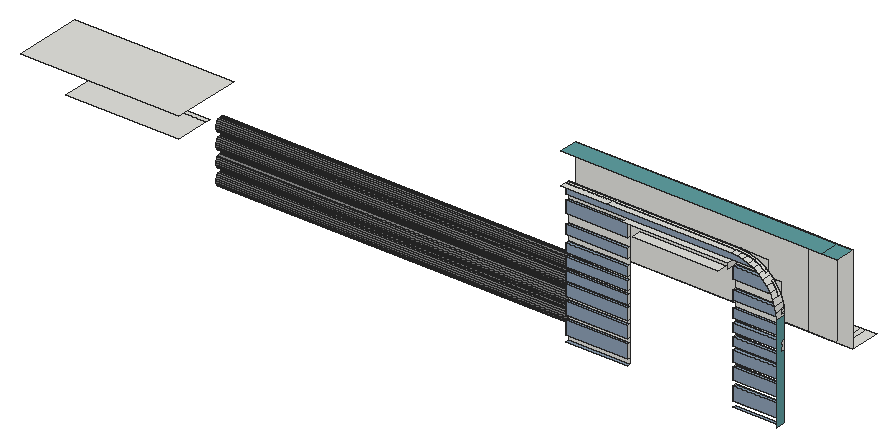
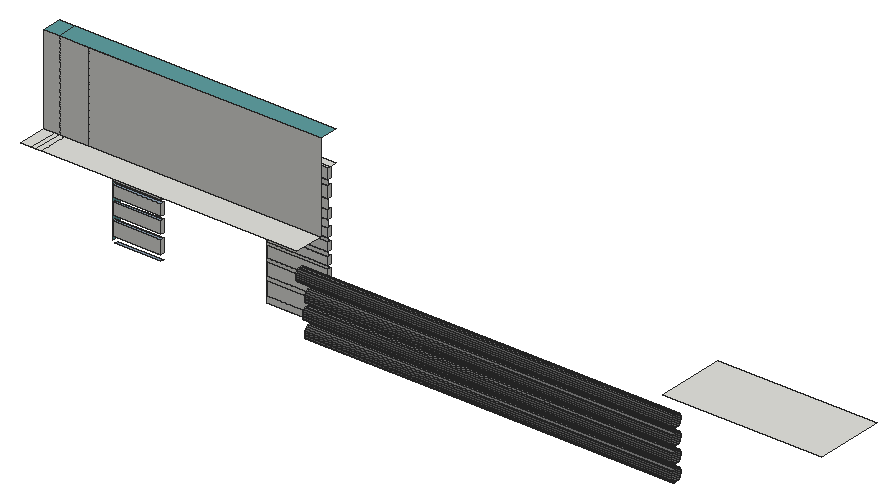
# SketchUp Ruby script. Lengths in inches.
U = 1.inch
M = Sketchup.active_model
def pt(a) = Geom::Point3d.new(a.map { |v| v * U })
def face(e, loops, mat)
  f = e.add_face(loops[0].map { |a| pt(a) })
  loops[1..].each { |l| e.add_face(l.map { |a| pt(a) }).erase! }
  f.material = f.back_material = mat if mat
  f
end
# faces: each face lists its corners as indices into pts; further lists are holes
def faces(e, pts, list, mat = nil) = list.each { |f| face(e, (f[0].is_a?(Array) ? f : [f]).map { |l| l.map { |i| pts[i] } }, mat) }
# xy, xz, yz: faces in a plane at the given z, y or x. An outline is a flat list of corners, or four numbers for a rectangle; further outlines are holes
def ring(l) = l.size == 4 ? [[l[0], l[1]], [l[2], l[1]], [l[2], l[3]], [l[0], l[3]]] : l.each_slice(2).to_a
def flat(e, list, mat, &to3) = list.each { |f| face(e, (f[0].is_a?(Array) ? f : [f]).map { |l| ring(l).map { |u, v| to3.(u, v) } }, mat) }
def xy(e, z, list, mat = nil) = flat(e, list, mat) { |x, y| [x, y, z] }
def xz(e, y, list, mat = nil) = flat(e, list, mat) { |x, z| [x, y, z] }
def yz(e, x, list, mat = nil) = flat(e, list, mat) { |y, z| [x, y, z] }
def lines(e, pts, list) = list.each { |a, b| e.add_line(pt(pts[a]), pt(pts[b])) }
# prism: a flat outline (further loops are holes) pulled along v
def prism(e, loops, v, mat = nil)
  f = face(e, loops, mat); d = Geom::Vector3d.new(v.map { |x| x * U })
  f.pushpull(f.normal.samedirection?(d) ? d.length : -d.length)
end
def box(e, o, s, mat = nil) = prism(e, [[o, [o[0] + s[0], o[1], o[2]], [o[0] + s[0], o[1] + s[1], o[2]], [o[0], o[1] + s[1], o[2]]]], [0, 0, s[2]], mat)
def at(x, y, z, deg = 0) = Geom::Transformation.translation(pt([x, y, z])) * Geom::Transformation.rotation(ORIGIN, Z_AXIS, deg.degrees)
def axes(o, x, y, z) = Geom::Transformation.new([*x, 0, *y, 0, *z, 0, *pt(o).to_a, 1])
def part(name) = M.definitions.add(name)
# library, detail: a bought-in or finely detailed component or shape, given as its bounding box
def library(name, o, s) = part(name).tap { |d| box(d.entities, o, s) }
def detail(e, o, s) = box(e.add_group.entities, o, s)
def put(e, d, t, mat = nil) = e.add_instance(d, t).tap { |i| i.material = mat if mat }
def group(e, t, mat = nil) = e.add_group.tap { |g| g.transformation = t; g.material = mat if mat }.entities
root = M.entities
M.materials.add("[0081_CadetBlue]").color = [95, 158, 160]
M.materials.add("[0110_LightSlateGray]").color = [139, 158, 178]
M.materials.add("[0133_Gray]").color = [128, 128, 128]
xy(root,388.02,[[160.53,8,179.47,9],[211.78,8,225.89,9]],"[0110_LightSlateGray]")
xy(root,389.79,[[160.53,8,179.47,9],[211.78,8,226.5625,9]],"[0110_LightSlateGray]")
xy(root,393.9,[[160.53,8,179.47,9],[211.78,8,226.5625,9]],"[0110_LightSlateGray]")
xy(root,395.43,[[160.53,8,179.47,9],[211.78,8,226.5625,9]],"[0110_LightSlateGray]")
xy(root,399.05,[[160.53,8,179.47,9],[211.78,8,226.5625,9]],"[0110_LightSlateGray]")
xy(root,400.39,[[160.53,8,179.47,9],[211.78,8,226.5625,9]],"[0110_LightSlateGray]")
xy(root,403.8125,[[160.53,8,179.47,9],[211.78,8,226.5625,9]],"[0110_LightSlateGray]")
xy(root,404.77,[[160.53,8,179.47,9],[211.78,8,226.5625,9]],"[0110_LightSlateGray]")
xy(root,407.32,[[160.53,8,179.47,9],[211.78,8,226.5625,9]],"[0110_LightSlateGray]")
xy(root,407.79,[[14,0,48.4375,10.4375],[14,10.4375,48.4375,12]])
xy(root,408.61,[[160.53,8,179.47,9],[211.78,8,226.59,9]],"[0110_LightSlateGray]")
xy(root,411.25,[[160.53,8,179.47,9],[211.78,8,226.59,9]],"[0110_LightSlateGray]")
xy(root,412.46,[[160.53,8,179.47,9],[211.78,8,226.5625,9]],"[0110_LightSlateGray]")
xy(root,414,[[0,0,48.4375,21],[160.53,12,238.75,21],[238.75,12,240.375,21],[240.375,12,241.9375,21],[241.9375,12,245.1875,21]])
xy(root,415.15,[[160.53,8,179.47,9],[211.78,8,226.5625,9]],"[0110_LightSlateGray]")
xy(root,417.42,[[160.53,8,179.47,9],[211.78,8,226.53,9]],"[0110_LightSlateGray]")
xy(root,420.17,[[160.53,8,179.47,9],[211.78,8,226.38,9]],"[0110_LightSlateGray]")
xy(root,423.16,[[160.53,8,179.47,9],[211.78,8,225.55,9]],"[0110_LightSlateGray]")
xy(root,425.29,[[182.53,6,208.72,9]])
xy(root,426.8,[[160.53,8,179.47,9],[211.78,8,223.28,9]],"[0110_LightSlateGray]")
xy(root,428.35,[[179.47,6,211.78,9]])
xy(root,428.36,[[160.53,8,221.7,9]],"[0110_LightSlateGray]")
xy(root,431.57,[[160.53,6,174.8,8],[174.8,6,212.95,8],[160.53,8,174.8,9],[174.8,8,212.95,9]])
xy(root,441.0625,[[160.53,6,240.375,12],[240.375,6,245.1875,12]],"[0081_CadetBlue]")
xz(root,8,[[160.53,389.79,179.47,393.9],[211.78,389.79,226.5625,393.9],[160.53,395.43,179.47,399.05],[211.78,395.43,226.5625,399.05],[160.53,400.39,179.47,403.8125],
  [211.78,400.39,226.5625,403.8125],[160.53,404.77,179.47,407.32],[211.78,404.77,226.5625,407.32],[160.53,408.61,179.47,411.25],[211.78,408.61,226.59,411.25],
  [160.53,412.46,179.47,415.15],[211.78,412.46,226.5625,415.15],[160.53,417.42,179.47,420.17],[211.78,417.42,226.53,417.42,226.53,418.83,226.47,419.72,226.38,420.17,211.78,420.17],[160.53,423.16,179.47,426.8],
  [211.78,423.16,225.55,423.16,224.76,424.76,223.77,426.24,223.28,426.8,211.78,426.8],[160.53,428.36,221.7,428.36,221.25,428.76,219.77,429.75,218.17,430.54,216.48,431.11,214.73,431.46,212.95,431.57,160.53,431.57]],"[0110_LightSlateGray]")
xz(root,9,[[160.53,388.02,179.47,389.79],[160.53,389.79,179.47,393.9],[211.78,389.79,226.5625,393.9],[160.53,393.9,179.47,395.43],[160.53,395.43,179.47,399.05],
  [211.78,395.43,226.5625,399.05],[160.53,399.05,179.47,400.39],[160.53,400.39,179.47,403.8125],[211.78,400.39,226.5625,403.8125],[160.53,403.8125,179.47,404.77],
  [160.53,404.77,179.47,407.32],[211.78,404.77,226.5625,407.32],[160.53,407.32,179.47,408.61],[160.53,408.61,179.47,411.25],[211.78,408.61,226.59,411.25],
  [160.53,411.25,179.47,412.46],[211.78,411.25,226.59,411.25,226.59,417.9375,226.53,418.83,226.53,417.42,211.78,417.42,211.78,415.15,226.5625,415.15,226.5625,412.46,211.78,412.46],[160.53,412.46,179.47,415.15],[211.78,412.46,226.5625,415.15],[160.53,415.15,179.47,417.42],
  [160.53,417.42,179.47,420.17],[211.78,417.42,211.78,420.17,226.38,420.17,226.47,419.72,226.53,418.83,226.53,417.42],[226.53,418.83,226.53,420.17,226.38,420.17,226.47,419.72],[160.53,420.17,179.47,423.16],[211.78,420.17,226.38,420.17,226.125,421.47,225.55,423.16,211.78,423.16],
  [160.53,423.16,179.47,426.8],[211.78,423.16,211.78,426.8,223.28,426.8,223.77,426.24,224.76,424.76,225.55,423.16],[225.55,423.16,225.55,426.8,223.28,426.8,223.77,426.24,224.76,424.76],[160.53,426.8,179.47,426.8,179.47,428.35,211.78,428.35,211.78,426.8,223.28,426.8,222.6,427.58,221.7,428.36,160.53,428.36],[160.53,428.36,160.53,431.57,212.95,431.57,214.73,431.46,216.48,431.11,218.17,430.54,219.77,429.75,221.25,428.76,221.7,428.36],
  [221.7,428.36,221.7,431.57,212.95,431.57,214.73,431.46,216.48,431.11,218.17,430.54,219.77,429.75,221.25,428.76]])
xz(root,12,[[160.53,414,231.375,441.0625],[231.375,414,240.375,441.0625],[240.375,414,245.1875,441.0625]])
yz(root,160.53,[[16.15,387.97,16.65,388.04,17.12,388.23,17.52,388.54,17.83,388.9375,18.02,389.41,18.09,389.91,18.02,390.41,17.83,390.875,17.52,391.28,17.12,391.59,16.65,391.78,16.15,391.84,15.65,391.78,15.18,391.59,14.78,391.28,14.47,390.875,14.28,390.41,14.22,389.91,14.28,389.41,14.47,388.9375,14.78,388.54,15.18,388.23,15.65,388.04],[8,389.79,9,393.9],[8,395.43,9,399.05],[16.15,397.84,16.65,397.91,17.12,398.1,17.52,398.41,17.83,398.8125,18.02,399.28,18.09,399.78,18.02,400.28,17.83,400.75,17.52,401.15,17.12,401.46,16.65,401.65,16.15,401.72,15.65,401.65,15.18,401.46,14.78,401.15,14.47,400.75,14.28,400.28,14.22,399.78,14.28,399.28,14.47,398.8125,14.78,398.41,15.18,398.1,15.65,397.91],[8,400.39,9,403.8125],
  [8,404.77,9,407.32],[8,408.61,9,411.25],[8,412.46,9,415.15],[8,417.42,9,420.17],[8,423.16,9,426.8],
  [8,428.36,9,431.57]])
yz(root,161.1875,[[16.15,392.91,16.65,392.97,17.12,393.17,17.52,393.47,17.83,393.875,18.02,394.34,18.09,394.84,18.02,395.35,17.83,395.8125,17.52,396.21,17.12,396.52,16.65,396.72,16.15,396.78,15.65,396.72,15.18,396.52,14.78,396.21,14.47,395.8125,14.28,395.35,14.22,394.84,14.28,394.34,14.47,393.875,14.78,393.47,15.18,393.17,15.65,392.97]])
yz(root,163.3125,[[16.15,402.78,16.65,402.85,17.12,403.04,17.52,403.35,17.83,403.75,18.02,404.22,18.09,404.72,18.02,405.22,17.83,405.6875,17.52,406.09,17.12,406.4,16.65,406.59,16.15,406.66,15.65,406.59,15.18,406.4,14.78,406.09,14.47,405.6875,14.28,405.22,14.22,404.72,14.28,404.22,14.47,403.75,14.78,403.35,15.18,403.04,15.65,402.85]])
yz(root,179.47,[[8,389.79,9,393.9],[8,395.43,9,399.05],[8,400.39,9,403.8125],[8,404.77,9,407.32],[8,408.61,9,411.25],
  [8,412.46,9,415.15],[8,417.42,9,420.17],[8,423.16,9,426.8]])
yz(root,211.78,[[8,389.79,9,393.9],[8,395.43,9,399.05],[8,400.39,9,403.8125],[8,404.77,9,407.32],[8,408.61,9,411.25],
  [8,412.46,9,415.15],[8,417.42,9,420.17],[8,423.16,9,426.8],[6,426.8,9,428.35]])
yz(root,226.53,[[8,417.42,9,418.83]])
yz(root,226.5625,[[8,389.79,9,393.9],[8,395.43,9,399.05],[8,400.39,9,403.8125],[8,404.77,9,407.32],[8,412.46,9,415.15]])
yz(root,226.59,[[8,408.61,9,411.25]])
yz(root,226.59,[[6,388.52,6,417.9375,9,417.9375,9,411.25,8,411.25,8,408.61,9,408.61,9,388.52]],"[0081_CadetBlue]")
p = [[48.4375,15.18,388.23],[48.4375,15.65,388.04],[160.53,15.65,388.04],[160.53,15.18,388.23],[48.4375,16.15,387.97],[160.53,16.15,387.97],
  [48.4375,16.65,388.04],[160.53,16.65,388.04],[48.4375,17.12,388.23],[160.53,17.12,388.23],[48.4375,14.78,388.54],[160.53,14.78,388.54],
  [48.4375,17.52,388.54],[160.53,17.52,388.54],[48.4375,14.48,388.9375],[160.53,14.47,388.9375],[48.4375,17.83,388.9375],[160.53,17.83,388.9375],
  [48.4375,14.28,389.41],[160.53,14.28,389.41],[48.4375,18.02,389.41],[160.53,18.02,389.41],[48.4375,14.22,389.91],[160.53,14.22,389.91],
  [48.4375,18.09,389.91],[160.53,18.09,389.91],[48.4375,14.28,390.41],[160.53,14.28,390.41],[48.4375,18.02,390.41],[160.53,18.02,390.41],
  [48.4375,14.48,390.875],[160.53,14.47,390.875],[48.4375,17.83,390.875],[160.53,17.83,390.875],[48.4375,14.78,391.28],[160.53,14.78,391.28],
  [48.4375,17.52,391.28],[160.53,17.52,391.28],[48.4375,15.18,391.59],[160.53,15.18,391.59],[48.4375,17.12,391.59],[160.53,17.12,391.59],
  [48.4375,15.65,391.78],[160.53,15.65,391.78],[48.4375,16.65,391.78],[160.53,16.65,391.78],[48.4375,16.15,391.84],[160.53,16.15,391.84],
  [48.4375,15.65,392.97],[48.4375,16.15,392.91],[161.1875,16.15,392.91],[161.1875,15.65,392.97],[48.4375,16.65,392.97],[161.1875,16.65,392.97],
  [48.4375,15.18,393.17],[161.1875,15.18,393.17],[48.4375,17.12,393.17],[161.1875,17.12,393.17],[48.4375,14.78,393.47],[161.1875,14.78,393.47],
  [48.4375,17.52,393.47],[161.1875,17.52,393.47],[48.4375,14.48,393.875],[161.1875,14.47,393.875],[48.4375,17.83,393.875],[161.1875,17.83,393.875],
  [48.4375,14.28,394.34],[161.1875,14.28,394.34],[48.4375,18.02,394.34],[161.1875,18.02,394.34],[48.4375,14.22,394.84],[161.1875,14.22,394.84],
  [48.4375,18.09,394.84],[161.1875,18.09,394.84],[48.4375,14.28,395.35],[161.1875,14.28,395.35],[48.4375,18.02,395.35],[161.1875,18.02,395.35],
  [48.4375,14.48,395.8125],[161.1875,14.47,395.8125],[48.4375,17.83,395.8125],[161.1875,17.83,395.8125],[48.4375,14.78,396.21],[161.1875,14.78,396.21],
  [48.4375,17.52,396.21],[161.1875,17.52,396.21],[48.4375,15.18,396.52],[161.1875,15.18,396.52],[48.4375,17.12,396.52],[161.1875,17.12,396.52],
  [48.4375,15.65,396.72],[161.1875,15.65,396.72],[48.4375,16.65,396.72],[161.1875,16.65,396.72],[48.4375,16.15,396.78],[161.1875,16.15,396.78],
  [48.4375,15.65,397.91],[48.4375,16.15,397.84],[160.53,16.15,397.84],[160.53,15.65,397.91],[48.4375,16.65,397.91],[160.53,16.65,397.91],
  [48.4375,15.18,398.1],[160.53,15.18,398.1],[48.4375,17.12,398.1],[160.53,17.12,398.1],[48.4375,14.78,398.41],[160.53,14.78,398.41],
  [48.4375,17.52,398.41],[160.53,17.52,398.41],[48.4375,14.48,398.8125],[160.53,14.47,398.8125],[48.4375,17.83,398.8125],[160.53,17.83,398.8125],
  [48.4375,14.28,399.28],[160.53,14.28,399.28],[48.4375,18.02,399.28],[160.53,18.02,399.28],[48.4375,14.22,399.78],[160.53,14.22,399.78],
  [48.4375,18.09,399.78],[160.53,18.09,399.78],[48.4375,14.28,400.28],[160.53,14.28,400.28],[48.4375,18.02,400.28],[160.53,18.02,400.28],
  [48.4375,14.48,400.75],[160.53,14.47,400.75],[48.4375,17.83,400.75],[160.53,17.83,400.75],[48.4375,14.78,401.15],[160.53,14.78,401.15],
  [48.4375,17.52,401.15],[160.53,17.52,401.15],[48.4375,15.18,401.46],[160.53,15.18,401.46],[48.4375,17.12,401.46],[160.53,17.12,401.46],
  [48.4375,15.65,401.65],[160.53,15.65,401.65],[48.4375,16.65,401.65],[160.53,16.65,401.65],[48.4375,16.15,401.72],[160.53,16.15,401.72],
  [48.4375,15.18,403.04],[48.4375,15.65,402.85],[163.3125,15.65,402.85],[163.3125,15.18,403.04],[48.4375,16.15,402.78],[163.3125,16.15,402.78],
  [48.4375,16.65,402.85],[163.3125,16.65,402.85],[48.4375,17.12,403.04],[163.3125,17.12,403.04],[48.4375,14.78,403.35],[163.3125,14.78,403.35],
  [48.4375,17.52,403.35],[163.3125,17.52,403.35],[48.4375,14.48,403.75],[163.3125,14.47,403.75],[48.4375,17.83,403.75],[163.3125,17.83,403.75],
  [48.4375,14.28,404.22],[163.3125,14.28,404.22],[48.4375,18.02,404.22],[163.3125,18.02,404.22],[48.4375,14.22,404.72],[163.3125,14.22,404.72],
  [48.4375,18.09,404.72],[163.3125,18.09,404.72],[48.4375,14.28,405.22],[163.3125,14.28,405.22],[48.4375,18.02,405.22],[163.3125,18.02,405.22],
  [48.4375,14.48,405.6875],[163.3125,14.47,405.6875],[48.4375,17.83,405.6875],[163.3125,17.83,405.6875],[48.4375,14.78,406.09],[163.3125,14.78,406.09],
  [48.4375,17.52,406.09],[163.3125,17.52,406.09],[48.4375,15.18,406.4],[163.3125,15.18,406.4],[48.4375,17.12,406.4],[163.3125,17.12,406.4],
  [48.4375,15.65,406.59],[163.3125,15.65,406.59],[48.4375,16.65,406.59],[163.3125,16.65,406.59],[48.4375,16.15,406.66],[163.3125,16.15,406.66],
  [226.53,9,418.83],[226.59,9,417.9375],[226.59,6,417.9375],[226.47,6,419.72],[226.47,8,419.72],[226.53,8,418.83],
  [226.47,9,419.72],[226.125,9,421.47],[226.38,9,420.17],[226.38,8,420.17],[226.125,6,421.47],[225.55,9,423.16],
  [225.55,6,423.16],[225.55,8,423.16],[224.76,6,424.76],[224.76,8,424.76],[224.76,9,424.76],[223.77,6,426.24],
  [223.77,8,426.24],[223.77,9,426.24],[222.6,9,427.58],[223.28,9,426.8],[223.28,8,426.8],[222.6,6,427.58],
  [221.7,9,428.36],[221.25,6,428.76],[221.25,8,428.76],[221.7,8,428.36],[221.25,9,428.76],[219.77,6,429.75],
  [219.77,8,429.75],[219.77,9,429.75],[218.17,6,430.54],[218.17,8,430.54],[218.17,9,430.54],[216.48,6,431.11],
  [216.48,8,431.11],[216.48,9,431.11],[214.73,6,431.46],[214.73,8,431.46],[214.73,9,431.46],[212.95,6,431.57],
  [212.95,8,431.57],[212.95,9,431.57]]
faces(root,p,[[0,1,2,3],[1,4,5,2],[4,6,7,5],[6,8,9,7],[10,0,3,11],[8,12,13,9],[14,10,11,15],[12,16,17,13],
  [18,14,15,19],[16,20,21,17],[22,18,19,23],[20,24,25,21],[26,22,23,27],[24,28,29,25],[30,26,27,31],[28,32,33,29],
  [34,30,31,35],[32,36,37,33],[38,34,35,39],[36,40,41,37],[42,38,39,43],[40,44,45,41],[46,42,43,47],[44,46,47,45],
  [48,49,50,51],[49,52,53,50],[54,48,51,55],[52,56,57,53],[58,54,55,59],[56,60,61,57],[62,58,59,63],[60,64,65,61],
  [66,62,63,67],[64,68,69,65],[70,66,67,71],[68,72,73,69],[74,70,71,75],[72,76,77,73],[78,74,75,79],[76,80,81,77],
  [82,78,79,83],[80,84,85,81],[86,82,83,87],[84,88,89,85],[90,86,87,91],[88,92,93,89],[94,90,91,95],[92,94,95,93],
  [96,97,98,99],[97,100,101,98],[102,96,99,103],[100,104,105,101],[106,102,103,107],[104,108,109,105],[110,106,107,111],[108,112,113,109],
  [114,110,111,115],[112,116,117,113],[118,114,115,119],[116,120,121,117],[122,118,119,123],[120,124,125,121],[126,122,123,127],[124,128,129,125],
  [130,126,127,131],[128,132,133,129],[134,130,131,135],[132,136,137,133],[138,134,135,139],[136,140,141,137],[142,138,139,143],[140,142,143,141],
  [144,145,146,147],[145,148,149,146],[148,150,151,149],[150,152,153,151],[154,144,147,155],[152,156,157,153],[158,154,155,159],[156,160,161,157],
  [162,158,159,163],[160,164,165,161],[166,162,163,167],[164,168,169,165],[170,166,167,171],[168,172,173,169],[174,170,171,175],[172,176,177,173],
  [178,174,175,179],[176,180,181,177],[182,178,179,183],[180,184,185,181],[186,182,183,187],[184,188,189,185],[190,186,187,191],[188,190,191,189]],"[0133_Gray]")
faces(root,p,[[192,193,194,195,196,197],[198,192,197,196],[199,200,201,196,195,202],[200,198,196,201],[203,199,202,204,205],[206,207,205,204],[208,203,205,207],[209,210,207,206],
  [211,208,207,210],[212,213,214,210,209,215],[213,211,210,214],[216,212,215,217,218,219],[220,216,219,218],[221,222,218,217],[223,220,218,222],[224,225,222,221],
  [226,223,222,225],[227,228,225,224],[229,226,225,228],[230,231,228,227],[232,229,228,231],[233,234,231,230],[235,232,231,234]])
